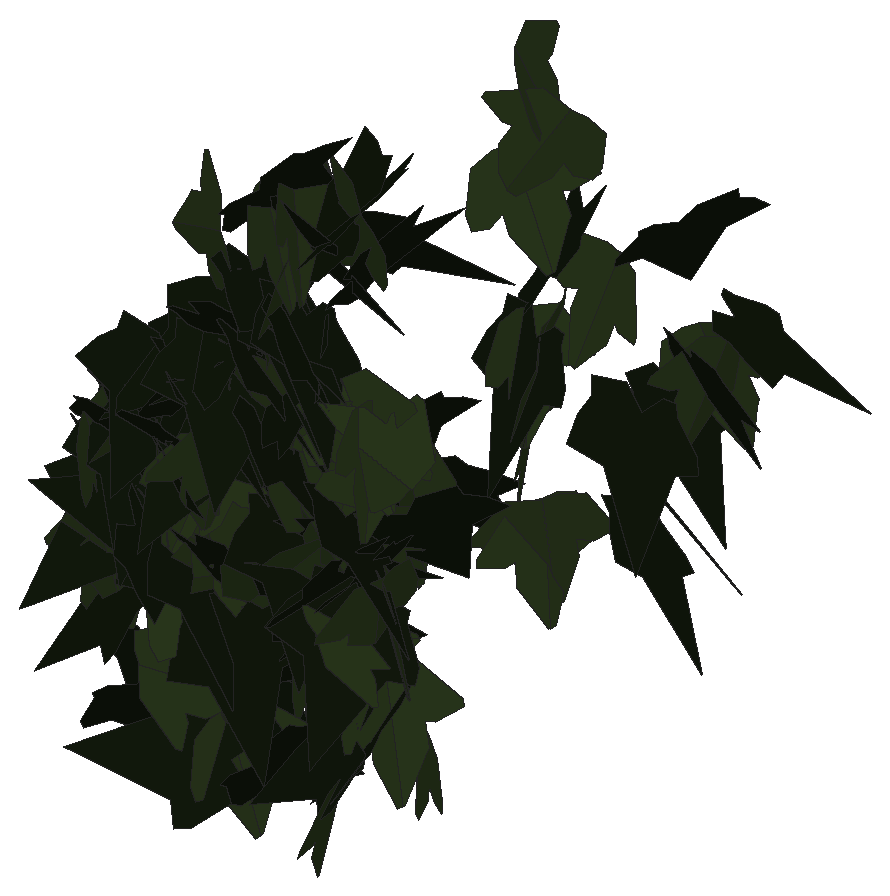
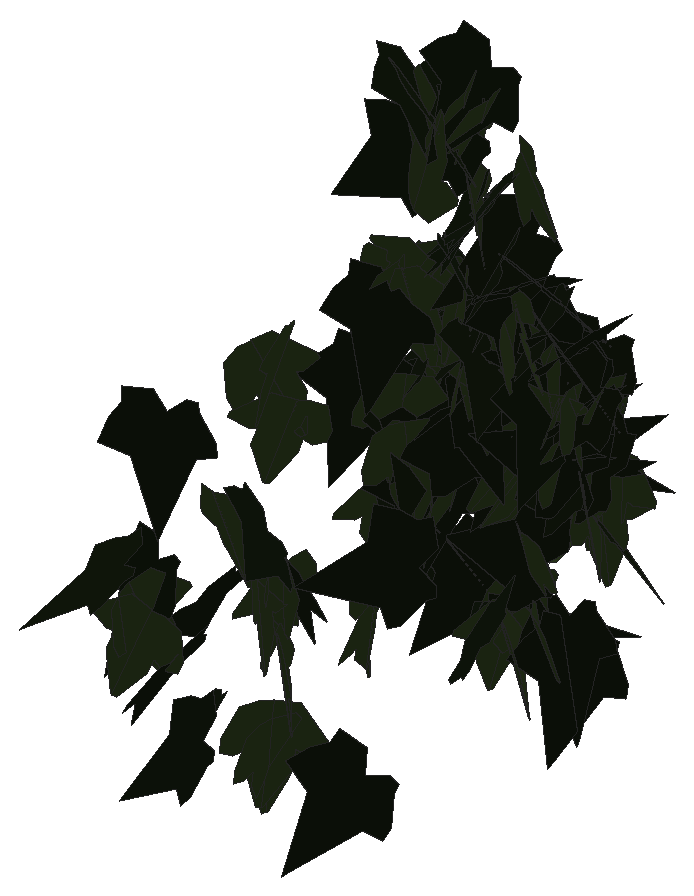
# SketchUp Ruby script. Lengths in inches.
U = 1.inch
M = Sketchup.active_model
def pt(a) = Geom::Point3d.new(a.map { |v| v * U })
def face(e, loops, mat)
  f = e.add_face(loops[0].map { |a| pt(a) })
  loops[1..].each { |l| e.add_face(l.map { |a| pt(a) }).erase! }
  f.material = f.back_material = mat if mat
  f
end
# faces: each face lists its corners as indices into pts; further lists are holes
def faces(e, pts, list, mat = nil) = list.each { |f| face(e, (f[0].is_a?(Array) ? f : [f]).map { |l| l.map { |i| pts[i] } }, mat) }
# xy, xz, yz: faces in a plane at the given z, y or x. An outline is a flat list of corners, or four numbers for a rectangle; further outlines are holes
def ring(l) = l.size == 4 ? [[l[0], l[1]], [l[2], l[1]], [l[2], l[3]], [l[0], l[3]]] : l.each_slice(2).to_a
def flat(e, list, mat, &to3) = list.each { |f| face(e, (f[0].is_a?(Array) ? f : [f]).map { |l| ring(l).map { |u, v| to3.(u, v) } }, mat) }
def xy(e, z, list, mat = nil) = flat(e, list, mat) { |x, y| [x, y, z] }
def xz(e, y, list, mat = nil) = flat(e, list, mat) { |x, z| [x, y, z] }
def yz(e, x, list, mat = nil) = flat(e, list, mat) { |y, z| [x, y, z] }
def lines(e, pts, list) = list.each { |a, b| e.add_line(pt(pts[a]), pt(pts[b])) }
# prism: a flat outline (further loops are holes) pulled along v
def prism(e, loops, v, mat = nil)
  f = face(e, loops, mat); d = Geom::Vector3d.new(v.map { |x| x * U })
  f.pushpull(f.normal.samedirection?(d) ? d.length : -d.length)
end
def box(e, o, s, mat = nil) = prism(e, [[o, [o[0] + s[0], o[1], o[2]], [o[0] + s[0], o[1] + s[1], o[2]], [o[0], o[1] + s[1], o[2]]]], [0, 0, s[2]], mat)
def at(x, y, z, deg = 0) = Geom::Transformation.translation(pt([x, y, z])) * Geom::Transformation.rotation(ORIGIN, Z_AXIS, deg.degrees)
def axes(o, x, y, z) = Geom::Transformation.new([*x, 0, *y, 0, *z, 0, *pt(o).to_a, 1])
def part(name) = M.definitions.add(name)
# library, detail: a bought-in or finely detailed component or shape, given as its bounding box
def library(name, o, s) = part(name).tap { |d| box(d.entities, o, s) }
def detail(e, o, s) = box(e.add_group.entities, o, s)
def put(e, d, t, mat = nil) = e.add_instance(d, t).tap { |i| i.material = mat if mat }
def group(e, t, mat = nil) = e.add_group.tap { |g| g.transformation = t; g.material = mat if mat }.entities
root = M.entities
M.materials.add("efeu1").color = [18, 25, 13]
M.materials.add("efeu2").color = [43, 57, 29]
c1 = part("ivyleaf_9")
p = [[1.54,2.16,1.25],[1.36,2.04,1.19],[-0.21,0.99,0.68],[-0.71,1.11,0.82],[-0.85,0.86,0.67],[-0.8,0.17,0.21],
  [-0.9,-0.01,0.1],[-0.67,-0.16,-0.02],[-0.08,-0.08,-0.05],[-0.03,-0.6,-0.4],[0.65,-0.88,-0.66],[0.83,-0.6,-0.49],
  [1.29,-0.42,-0.43],[1.8125,-0.07,-0.26],[1.21,0.44,0.15]]
faces(c1.entities,p,[[0,1,2,3,4,5,6,7,8,9,10,11,12,13,14]],"efeu1")
c2 = part("ivyleaf_10")
p = [[0,0.5,-0.03],[-0.0625,2.02,-0.43],[-0.19,2.01,-0.46],[-0.54,1.05,-0.29],[-0.52,0.625,-0.18],[-0.83,0.76,-0.28],
  [-1.16,0.64,-0.33],[-1.15,0.33,-0.24],[-0.77,-0.39,0.02],[-0.3,-0.51,0.16],[0.04,-0.48,0.23],[-0.02,2.01,-0.4375],
  [-0.06,2.01,-0.43],[0.04,-0.49,0.23],[0.67,-0.49,0.14],[1.38,0.36,-0.2],[1.375,0.51,-0.24],[0.81,0.65,-0.19],
  [0.62,0.59,-0.15],[0.6,1.09,-0.28],[0.5,1.23,-0.31]]
faces(c2.entities,p,[[0,1,2,3,4,5,6,7,8,9,10],[11,12,0,13,14,15,16,17,18,19,20]],"efeu2")
put(root,c1,axes([50.83,221.67,248.625],[0.1935,0.41398,0.20293],[0.05928,0.19591,-0.45619],[-0.45721,0.20061,0.02674]))
put(root,c2,axes([49.97,222.09,245.54],[-0.1538,-0.4756,0.0121],[-0.00834,-0.01002,-0.49983],[0.47568,-0.15395,-0.00486]))
put(root,c1,axes([49.07,221.8,245.6],[0.41212,0.2285,-0.16718],[-0.1986,0.02289,-0.45829],[-0.20179,0.44414,0.10963]))
put(root,c2,axes([48.77,222.02,244.17],[-0.48717,-0.10879,-0.02873],[0.02886,0.0026,-0.49916],[0.10875,-0.48801,0.00375]))
put(root,c1,axes([49.25,221.88,244.47],[0.34024,-0.20161,-0.30593],[-0.18932,0.2607,-0.38235],[0.31368,0.37602,0.10106]))
put(root,c1,axes([49.95,222.35,246.25],[-0.16434,-0.47191,-0.01723],[0.10804,-0.01981,-0.48779],[0.4597,-0.16405,0.10848]))
put(root,c1,axes([48.94,222.12,243.71],[-0.43937,0.23681,-0.02957],[0.02566,-0.0147,-0.49912],[-0.23726,-0.44012,0.00076]))
put(root,c2,axes([51.3,222.1,242.4],[0.16319,-0.46581,-0.07995],[-0.02665,0.07538,-0.49357],[0.47187,0.16536,-0.00022]))
put(root,c1,axes([49.05,222.46,245.79],[-0.1501,-0.44035,0.18319],[0.02153,-0.19811,-0.45857],[0.47645,-0.12978,0.07844]))
put(root,c1,axes([49.54,222.27,244.13],[0.17959,-0.466,0.02431],[0.01363,-0.0208,-0.49938],[0.46644,0.18003,0.00523]))
put(root,c2,axes([50.65,222.03,248.23],[-0.04152,0.49815,0.01122],[-0.00034,0.01123,-0.49987],[-0.49827,-0.04152,-0.00059]))
put(root,c1,axes([50.1,222.19,243.67],[-0.26055,-0.20397,-0.37484],[0.32141,0.19512,-0.32958],[0.28073,-0.4127,0.02944]))
put(root,c1,axes([48.8,222.44,244.37],[-0.41848,-0.24744,0.11682],[-0.04802,-0.14374,-0.47648],[0.26938,-0.41002,0.09654]))
put(root,c2,axes([50.84,222.15,248.38],[-0.07259,0.48061,-0.11725],[0.00929,-0.11716,-0.48599],[-0.49462,-0.07273,0.00808]))
put(root,c1,axes([48.71,222.21,245.32],[0.13712,0.00671,-0.48078],[0.47258,0.09032,0.13604],[0.08868,-0.49173,0.01843]))
put(root,c1,axes([49.31,222.39,244.3],[-0.12662,-0.00035,0.4837],[-0.46323,-0.14385,-0.12136],[0.13925,-0.47886,0.03611]))
put(root,c1,axes([49.85,222.29,246.5625],[-0.48958,0.10147,0.00322],[-0.01668,-0.06475,-0.49551],[-0.10015,-0.48529,0.06679]))
put(root,c2,axes([48.64,222,245.21],[-0.10951,0.46063,0.1607],[-0.10515,0.13854,-0.46878],[-0.47639,-0.13647,0.06653]))
put(root,c2,axes([50.59,222.24,247.41],[0.24806,-0.43367,-0.02004],[0.0197,0.0343,-0.49843],[0.43368,0.24649,0.03411]))
put(root,c1,axes([51.33,222.46,244.05],[-0.22075,-0.44849,0.01137],[-0.02142,-0.00213,-0.49954],[0.44812,-0.22103,-0.01827]))
put(root,c1,axes([48.84,222.48,245.04],[-0.07595,-0.48881,0.07277],[-0.00157,-0.07338,-0.49458],[0.4942,-0.07535,0.00961]))
put(root,c1,axes([49.9375,221.98,246.86],[0.49067,0.07003,0.06584],[0.05406,0.08213,-0.49024],[-0.07948,0.48821,0.07302]))
put(root,c1,axes([49.69,222.47,245.58],[-0.36573,-0.34085,0.00764],[-0.00655,-0.00418,-0.49994],[0.34088,-0.36579,-0.00141]))
put(root,c2,axes([49.98,222.05,247.75],[-0.14713,0.11817,0.46302],[-0.45263,0.12088,-0.17468],[-0.15322,-0.47056,0.0714]))
put(root,c1,axes([50.72,222.14,248.04],[0.4811,-0.11076,0.07921],[0.07481,-0.02801,-0.49358],[0.11378,0.48677,-0.01038]))
put(root,c2,axes([51.71,222.36,245.74],[0.21815,0.26843,0.36105],[-0.22777,-0.28014,0.34589],[0.38798,-0.31539,0.00005]))
put(root,c1,axes([50.7,222.46,246.87],[0.10866,-0.47833,0.09693],[0.04469,-0.08914,-0.48996],[0.486,0.11515,0.02338]))
put(root,c2,axes([50.47,222.21,244.12],[-0.2112,-0.38074,0.24584],[0.24065,0.13561,0.41677],[-0.38404,0.29436,0.12597]))
put(root,c1,axes([49.81,222.05,244.39],[0.47717,0.0885,-0.12032],[-0.12216,-0.00054,-0.48485],[-0.08595,0.49211,0.0211]))
put(root,c1,axes([50.46,222.41,247],[0.17622,-0.4673,0.024],[0.00527,-0.02367,-0.49941],[0.46789,0.17626,-0.00342]))
put(root,c1,axes([51.37,222.24,242.9],[-0.42963,0.25021,0.05298],[-0.04575,0.02672,-0.49718],[-0.25164,-0.43206,-0.00007]))
put(root,c1,axes([50.66,222.25,246.98],[0.36834,-0.32508,-0.09301],[-0.077,0.05329,-0.49115],[0.32924,0.37614,-0.01081]))
put(root,c2,axes([49.75,222.29,245.17],[0.32723,0.33177,-0.18123],[-0.19104,-0.06172,-0.45793],[-0.32622,0.36894,0.08637]))
put(root,c2,axes([49.37,221.97,243.01],[0.29741,-0.30234,-0.26484],[0.242,0.39774,-0.18232],[0.32092,-0.01973,0.38291]))
put(root,c1,axes([50.86,222.26,246.42],[-0.41952,0.26867,-0.04263],[0.041,-0.01501,-0.49809],[-0.26893,-0.42141,-0.00943]))
put(root,c1,axes([50.16,222.32,246.54],[0.35503,-0.35201,-0.0063],[0.00055,0.0095,-0.49991],[0.35207,0.35496,0.00713]))
put(root,c1,axes([51.61,222.04,248.47],[-0.1084,0.47526,0.11124],[-0.09395,0.0915,-0.48249],[-0.47898,-0.12551,0.06946]))
put(root,c1,axes([50.26,222.29,247.35],[0.29833,-0.389,-0.09836],[0.01101,0.13046,-0.48255],[0.4011,0.28575,0.08641]))
put(root,c2,axes([48.61,222.31,243.93],[-0.10159,-0.48929,-0.01666],[0.00579,0.01581,-0.49972],[0.48954,-0.10173,0.00245]))
put(root,c1,axes([49.41,222.4,245.94],[0.31038,-0.37724,0.10655],[0.09114,-0.06273,-0.4876],[0.38126,0.32211,0.02982]))
put(root,c1,axes([50.57,222.53,244.62],[-0.0174,-0.49965,-0.00661],[0.00029,0.0066,-0.49996],[0.4997,-0.01741,0.00006]))
put(root,c1,axes([51.125,222.45,245.02],[0.28134,-0.40471,0.08399],[0.05613,-0.06325,-0.4928],[0.40951,0.28672,0.00984]))
put(root,c2,axes([49.11,222.44,245.18],[-0.12917,0.40257,-0.26694],[0.08585,-0.25279,-0.42276],[-0.47534,-0.15505,-0.00381]))
put(root,c1,axes([49.8125,222.1,246.1],[0.17652,0.46206,-0.07305],[-0.0442,-0.06125,-0.49426],[-0.46571,0.18096,0.01922]))
put(root,c2,axes([50.21,222.27,246.26],[-0.4988,0.03323,0.00949],[-0.00945,0.00088,-0.49991],[-0.03324,-0.49889,-0.00025]))
put(root,c1,axes([49.73,222.48,242.04],[-0.33562,0.05192,0.36696],[-0.37061,-0.04989,-0.3319],[0.00215,-0.49479,0.07197]))
put(root,c2,axes([49.6,222.21,243.78],[0.32605,0.26622,0.26984],[0.20562,0.1748,-0.42091],[-0.31844,0.38545,0.0045]))
put(root,c2,axes([51.52,222.2,248.28],[-0.32838,0.11619,0.3587],[-0.34935,0.08519,-0.34742],[-0.14185,-0.47879,0.02524]))
put(root,c1,axes([50.31,222.3,245.82],[0.36662,-0.3118,-0.13554],[-0.08986,0.10336,-0.48087],[0.32789,0.37696,0.01975]))
put(root,c1,axes([49.34,222.41,245.97],[-0.45896,0.19267,-0.04725],[0.04936,-0.00442,-0.49754],[-0.19214,-0.46137,-0.01496]))
put(root,c2,axes([49.41,222.58,245.4375],[0.209,-0.25403,-0.37655],[0.2425,-0.28808,0.32894],[-0.38407,-0.32012,0.00278]))
put(root,c2,axes([49.41,222.41,245.59],[-0.42163,0.21691,-0.15869],[0.10658,-0.13608,-0.46917],[-0.24672,-0.42946,0.06852]))
put(root,c2,axes([51.57,222.4,244.4],[-0.07434,-0.49229,-0.04603],[0.00187,0.04627,-0.49785],[0.49444,-0.0742,-0.00504]))
put(root,c1,axes([51.44,222.23,248.34],[-0.29725,0.33126,0.22783],[-0.15403,0.16788,-0.44507],[-0.37137,-0.33478,0.00224]))
put(root,c2,axes([50.52,222.58,244.94],[-0.12247,0.04423,-0.48275],[0.36852,-0.315,-0.12235],[-0.31496,-0.38577,0.04456]))
put(root,c2,axes([51.51,222.47,246.04],[0.07891,0.46927,-0.15348],[-0.03458,-0.14979,-0.47578],[-0.49252,0.0857,0.00881]))
put(root,c1,axes([51.05,222.02,244.35],[0.16587,0.39709,0.25457],[0.07874,0.24275,-0.42997],[-0.46507,0.18273,0.018]))
put(root,c1,axes([48.32,222.58,244.49],[0.26609,-0.27358,0.32303],[0.22547,-0.23133,-0.38164],[0.35827,0.34877,0.00026]))
put(root,c2,axes([51.3,222.09,244],[0.37285,-0.20389,-0.26346],[0.18484,0.45558,-0.09099],[0.27716,-0.02954,0.4151]))
put(root,c2,axes([48.79,222.48,245.18],[0.02448,-0.49933,-0.00811],[-0.00614,0.00781,-0.4999],[0.49936,0.02457,-0.00575]))
put(root,c2,axes([51.21,222.41,246.19],[0.39918,0.11783,0.27708],[0.26659,0.07556,-0.4162],[-0.13995,0.48001,-0.0025]))
put(root,c1,axes([51.59,222.35,242.99],[-0.28937,0.40651,-0.03183],[0.01736,-0.02671,-0.49898],[-0.40739,-0.28988,0.00134]))
put(root,c2,axes([49.73,222.56,245.77],[0.14432,-0.47362,0.06971],[0.0151,-0.06827,-0.49509],[0.47848,0.14501,-0.0054]))
put(root,c2,axes([49.25,222.45,244.46],[0.47008,-0.17034,-0.00285],[0.02819,0.08601,-0.49174],[0.16802,0.46215,0.09047]))
put(root,c2,axes([48.8125,222.64,244.59],[-0.18634,-0.42398,0.18848],[0.04849,-0.21979,-0.44648],[0.46144,-0.14811,0.12303]))
put(root,c2,axes([50.71,222.52,243.375],[-0.09021,0.48731,-0.06628],[0.00748,-0.06602,-0.49557],[-0.49174,-0.0904,0.00462]))
put(root,c1,axes([48.64,222.38,245.43],[0.49469,-0.01943,-0.07],[-0.06886,0.02811,-0.49444],[0.02315,0.49883,0.02513]))
put(root,c1,axes([50.45,222.18,242.38],[0.24309,0.38406,0.20834],[0.11088,0.17639,-0.45452],[-0.42263,0.26718,0.00059]))
put(root,c2,axes([49.68,222.33,244.3],[-0.17504,-0.28095,-0.37474],[0.22779,0.29848,-0.33018],[0.40923,-0.28631,0.02351]))
put(root,c2,axes([51.3125,222.52,245.94],[0.43502,0.22007,-0.11105],[-0.15855,0.07734,-0.46784],[-0.18874,0.44225,0.13708]))
put(root,c2,axes([49.07,222.61,245.14],[0.49748,0.04692,0.01754],[0.01721,0.00432,-0.49968],[-0.04704,0.49778,0.00269]))
put(root,c2,axes([49.6875,222.66,242.43],[-0.24925,-0.12009,0.41648],[-0.37664,-0.17775,-0.27667],[0.2145,-0.45165,-0.00185]))
put(root,c2,axes([50.64,222.47,246.21],[-0.38915,0.30332,0.08096],[-0.07389,0.03683,-0.49314],[-0.30512,-0.39578,0.01616]))
put(root,c2,axes([51.51,222.56,244.34],[-0.30982,0.38386,-0.08161],[0.04878,-0.0655,-0.49329],[-0.3894,-0.31362,0.00314]))
put(root,c1,axes([48.64,222.7,244.36],[0.34656,-0.31437,0.17627],[0.15071,-0.09573,-0.46704],[0.32739,0.37684,0.0284]))
put(root,c2,axes([49.67,222.29,243.99],[0.10018,-0.18485,-0.45365],[0.10146,0.46083,-0.16536],[0.47924,-0.05892,0.12984]))
put(root,c2,axes([50.53,222.54,244.95],[-0.19792,0.44642,-0.10739],[-0.03587,0.10156,0.48826],[0.45776,0.20098,-0.00817]))
put(root,c2,axes([50.97,222.58,243.41],[-0.34564,0.35801,0.04864],[-0.08644,-0.01659,-0.49219],[-0.3508,-0.34865,0.07336]))
put(root,c1,axes([50.43,222.54,244.85],[0.12657,0.19591,-0.44226],[-0.44602,-0.12966,-0.18508],[-0.18721,0.44137,0.14194]))
put(root,c1,axes([49.17,222.71,243.11],[0.30632,-0.14744,0.36665],[0.33742,-0.1439,-0.33976],[0.20571,0.45558,0.01134]))
put(root,c2,axes([51.5,222.65,243.2],[0.18065,0.46586,0.0185],[0.00811,0.0167,-0.49966],[-0.46616,0.18082,-0.00152]))
put(root,c1,axes([50.95,222.5,243.625],[0.18723,0.45907,-0.06484],[-0.02936,-0.05805,-0.49575],[-0.46269,0.18944,0.00522]))
put(root,c2,axes([48.51,222.71,244.24],[0.21389,-0.41991,-0.1671],[-0.07739,0.1481,-0.47125],[0.44526,0.22746,-0.00164]))
put(root,c1,axes([48.62,222.71,244.48],[0.23842,-0.06111,0.43523],[0.42045,-0.11247,-0.24611],[0.12798,0.48334,-0.00224]))
put(root,c2,axes([49.31,222.79,243.23],[0.40825,-0.28103,-0.06602],[-0.03666,0.06296,-0.49466],[0.28634,0.40873,0.0308]))
put(root,c2,axes([49.71,222.65,242.17],[0.15937,0.46063,0.11145],[-0.00049,0.11775,-0.48594],[-0.47392,0.15478,0.03799]))
put(root,c1,axes([49.15,222.4375,245.11],[0.14162,0.46104,0.13187],[0.02926,0.12894,-0.4822],[-0.47863,0.14429,0.00954]))
put(root,c1,axes([50.14,222.42,245.48],[0.03156,0.4359,0.2429],[-0.06147,0.24492,-0.43155],[-0.4952,-0.00262,0.06905]))
put(root,c1,axes([51.375,222.36,247.63],[0.19353,0.23542,0.39639],[0.14208,0.37852,-0.29417],[-0.43859,0.2265,0.07961]))
put(root,c1,axes([50.28,222.66,244.29],[0.34387,-0.07711,0.3547],[0.36251,0.04797,-0.34101],[0.01856,0.49168,0.08889]))
put(root,c2,axes([50.86,222.83,247.53],[-0.44667,0.21925,-0.04915],[-0.04242,0.02513,0.49756],[0.22065,0.44866,-0.00385]))
put(root,c1,axes([51.14,222.53,244.27],[0.02648,0.48296,0.1267],[0.00056,0.12685,-0.48364],[-0.4993,0.02576,0.00617]))
put(root,c2,axes([51.12,222.89,244.7],[-0.36243,-0.34057,-0.05151],[0.02776,0.04565,-0.49714],[0.34332,-0.36322,-0.01418]))
put(root,c1,axes([48.66,222.86,242.55],[0.30847,0.16759,-0.35604],[-0.32064,-0.1552,-0.35086],[-0.22811,0.44478,0.01172]))
put(root,c2,axes([48.89,223.09,242.41],[0.34527,-0.36039,0.03011],[0.01711,-0.0253,-0.49907],[0.36124,0.34566,-0.00514]))
put(root,c2,axes([50.93,223.06,244.2],[-0.30562,-0.39307,0.04577],[-0.02793,-0.03626,-0.4979],[0.39474,-0.30689,0.00021]))
put(root,c1,axes([51.42,222.76,245.875],[0.12954,0.48256,0.01882],[-0.0013,0.01983,-0.4996],[-0.48293,0.12939,0.00639]))
put(root,c1,axes([48.51,222.8125,242.21],[0.21092,0.45317,-0.01226],[-0.00121,-0.01296,-0.49983],[-0.45333,0.21088,-0.00437]))
put(root,c1,axes([51.5,222.94,244.94],[0.27506,0.41746,-0.00817],[-0.0029,-0.00787,-0.49993],[-0.41753,0.27507,-0.00191]))
put(root,c2,axes([49.15,223.35,242.37],[0.29478,-0.40199,-0.03881],[-0.02611,0.02897,-0.49848],[0.40301,0.29591,-0.00391]))
put(root,c1,axes([49.36,223.65,242.33],[0.07835,-0.35639,0.34183],[0.10562,-0.326,-0.36409],[0.4824,0.12926,0.0242]))
put(root,c2,axes([51.25,223.47,242.33],[-0.34071,0.31326,0.18917],[-0.21537,0.03732,-0.44969],[-0.29586,-0.38791,0.1095]))
put(root,c2,axes([49.51,225.52,243.55],[-0.10972,0.46585,-0.14473],[0.01864,-0.14423,-0.47838],[-0.48746,-0.11037,0.01429]))
put(root,c2,axes([50.37,226.48,247.01],[-0.36356,-0.1957,0.28201],[-0.22044,-0.18176,-0.41033],[0.26311,-0.42269,0.04588]))
put(root,c1,axes([49.94,226.65,244.54],[-0.41865,-0.01636,-0.27288],[0.27233,0.01849,-0.41892],[0.0238,-0.49939,-0.00657]))
put(root,c2,axes([49.96,226.41,246.42],[0.31804,0.35248,0.15686],[0.08664,0.13285,-0.47418],[-0.37596,0.3288,0.02342]))
put(root,c1,axes([48.07,226.49,245.0625],[0.4151,-0.02202,0.27787],[0.27845,0.05562,-0.41155],[-0.01279,0.49641,0.05844]))
put(root,c2,axes([49.97,226.5625,247.43],[-0.214,0.40888,0.1924],[-0.07781,0.17636,-0.46135],[-0.44514,-0.2274,-0.01185]))
put(root,c2,axes([49.77,226.83,244.48],[0.11443,0.47965,-0.08271],[-0.03353,-0.077,-0.4929],[-0.48557,0.11835,0.01454]))
put(root,c1,axes([50.83,227.08,243.89],[-0.00013,-0.49897,0.03211],[-0.00636,-0.03211,-0.49893],[0.49996,-0.00054,-0.00634]))
put(root,c2,axes([49.97,226.65,244.23],[0.07755,-0.34739,-0.35115],[-0.04587,0.34885,-0.35525],[0.49182,0.08731,0.02223]))
put(root,c2,axes([49.64,226.97,243.59],[0.28862,-0.40491,-0.0524],[0.01643,0.07563,-0.49397],[0.40796,0.28342,0.05696]))
put(root,c2,axes([49.83,226.96,242.58],[-0.3544,-0.34939,-0.04826],[0.04405,0.02402,-0.49748],[0.34994,-0.35686,0.01376]))
put(root,c2,axes([49.72,227.07,242.44],[-0.14653,-0.47774,0.01713],[0.15556,-0.0646,-0.47077],[0.45203,-0.13264,0.16757]))
put(root,c2,axes([50.46,227.04,245.25],[0.46762,-0.15072,-0.09282],[-0.08519,0.03818,-0.49121],[0.15516,0.47521,0.01002]))
put(root,c1,axes([51.38,226.98,246.13],[0.10888,0.48542,-0.05016],[-0.03994,-0.04235,-0.4966],[-0.48636,0.11215,0.02955]))
put(root,c2,axes([49.74,227.25,244.56],[0.14197,-0.43912,-0.19241],[-0.05256,0.18521,-0.46145],[0.47653,0.15125,0.00643]))
put(root,c1,axes([48.375,227.09,242.41],[0.43063,0.25208,0.03193],[0.0174,0.03344,-0.49858],[-0.25349,0.43051,0.02003]))
put(root,c1,axes([49.88,226.98,245.12],[0.053,0.28577,0.40685],[-0.08619,0.40824,-0.27552],[-0.48966,-0.04093,0.09253]))
put(root,c1,axes([50.48,227.55,242.4375],[0.25853,-0.42329,0.06314],[0.04147,-0.04864,-0.4959],[0.42596,0.26165,0.00996]))
put(root,c1,axes([51.18,227.43,244.43],[0.45128,0.00521,-0.21521],[-0.21527,0.00825,-0.45121],[-0.00115,0.4999,0.00969]))
put(root,c2,axes([51.02,227.93,244.2],[-0.07573,-0.46691,0.16205],[-0.00149,-0.16373,-0.47243],[0.49423,-0.07204,0.0234]))
put(root,c1,axes([50.47,228.04,243.61],[0.17114,-0.45878,-0.10117],[-0.02762,0.09767,-0.48959],[0.46899,0.17316,0.00808]))
put(root,c1,axes([50.06,228,242.7],[0.45572,-0.20357,0.02965],[0.02569,-0.01519,-0.49911],[0.20411,0.45643,-0.00339]))
put(root,c1,axes([51.25,228,244.63],[0.44602,-0.20354,-0.09819],[-0.00327,0.21141,-0.4531],[0.22596,0.40482,0.18725]))
put(root,c2,axes([50.73,228.15,244.08],[0.44941,0.08617,0.2015],[0.15596,0.19723,-0.43218],[-0.15397,0.45131,0.15039]))
